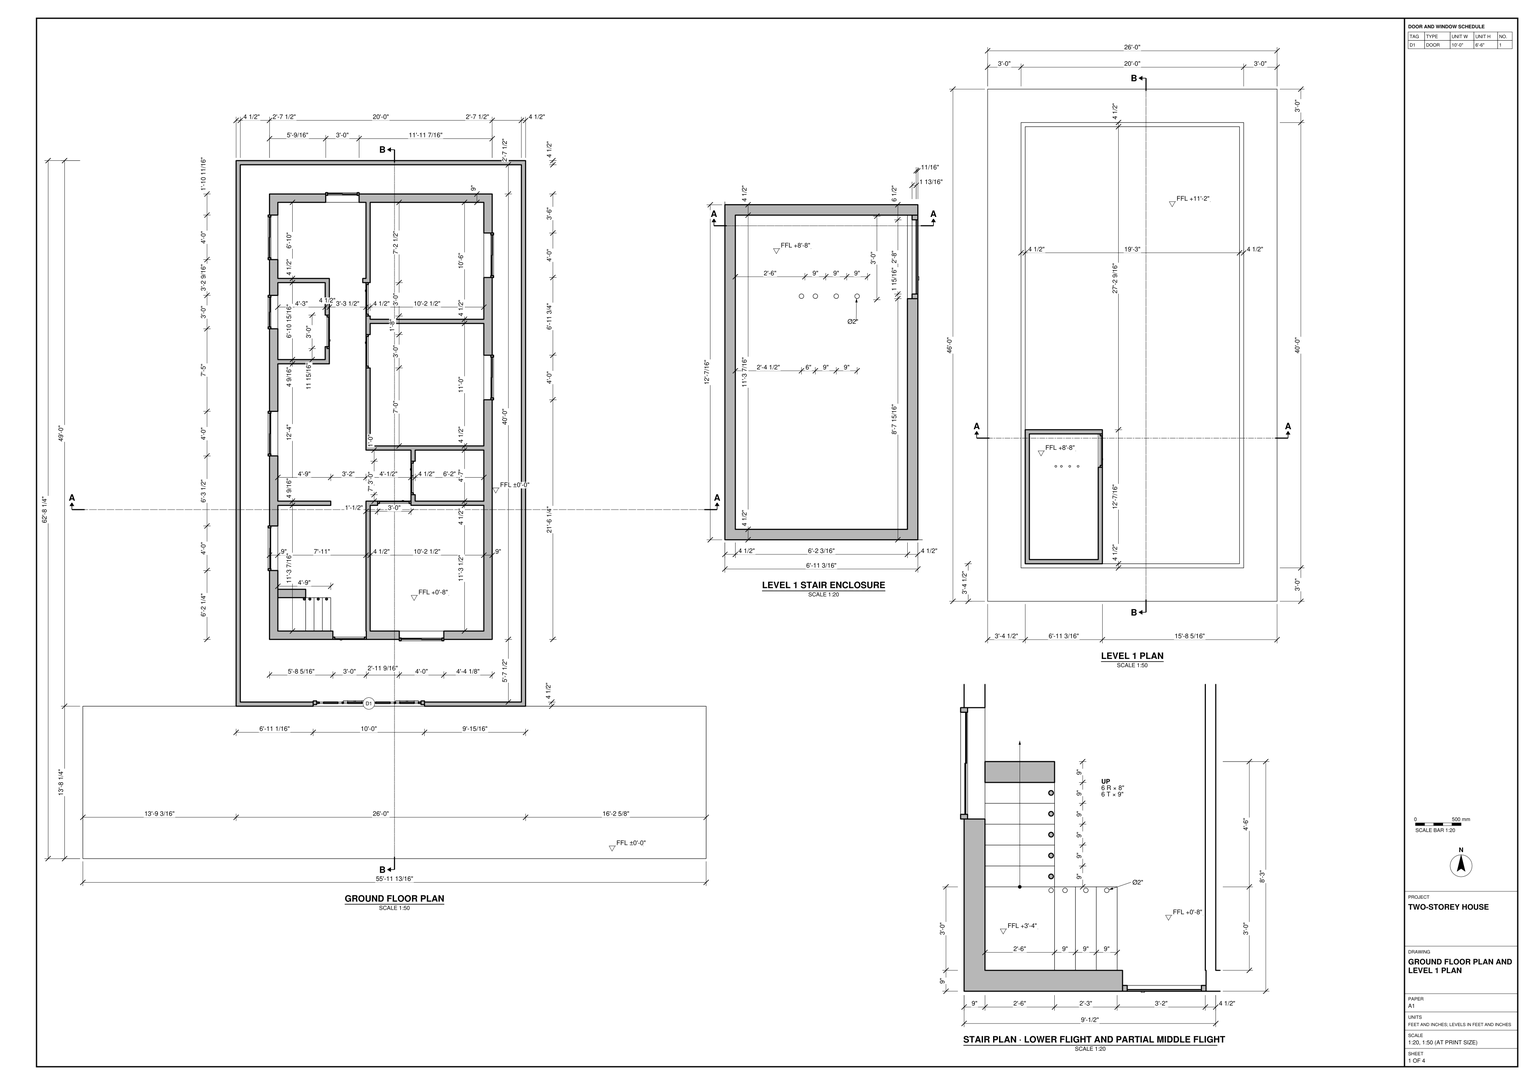
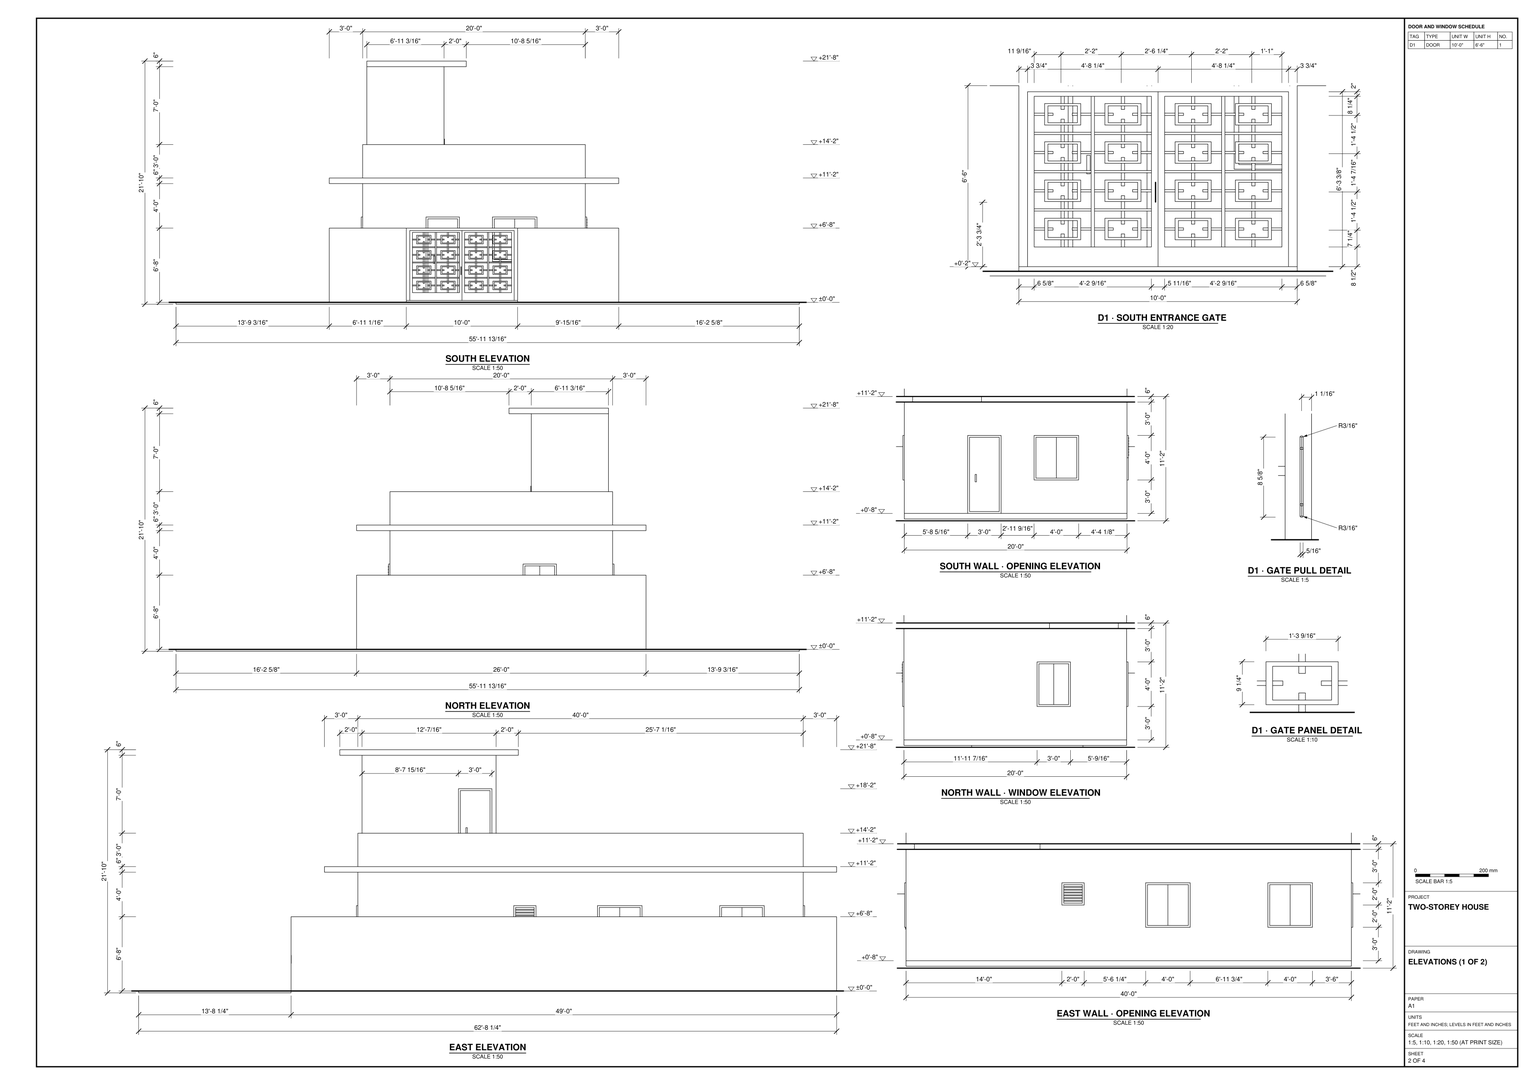
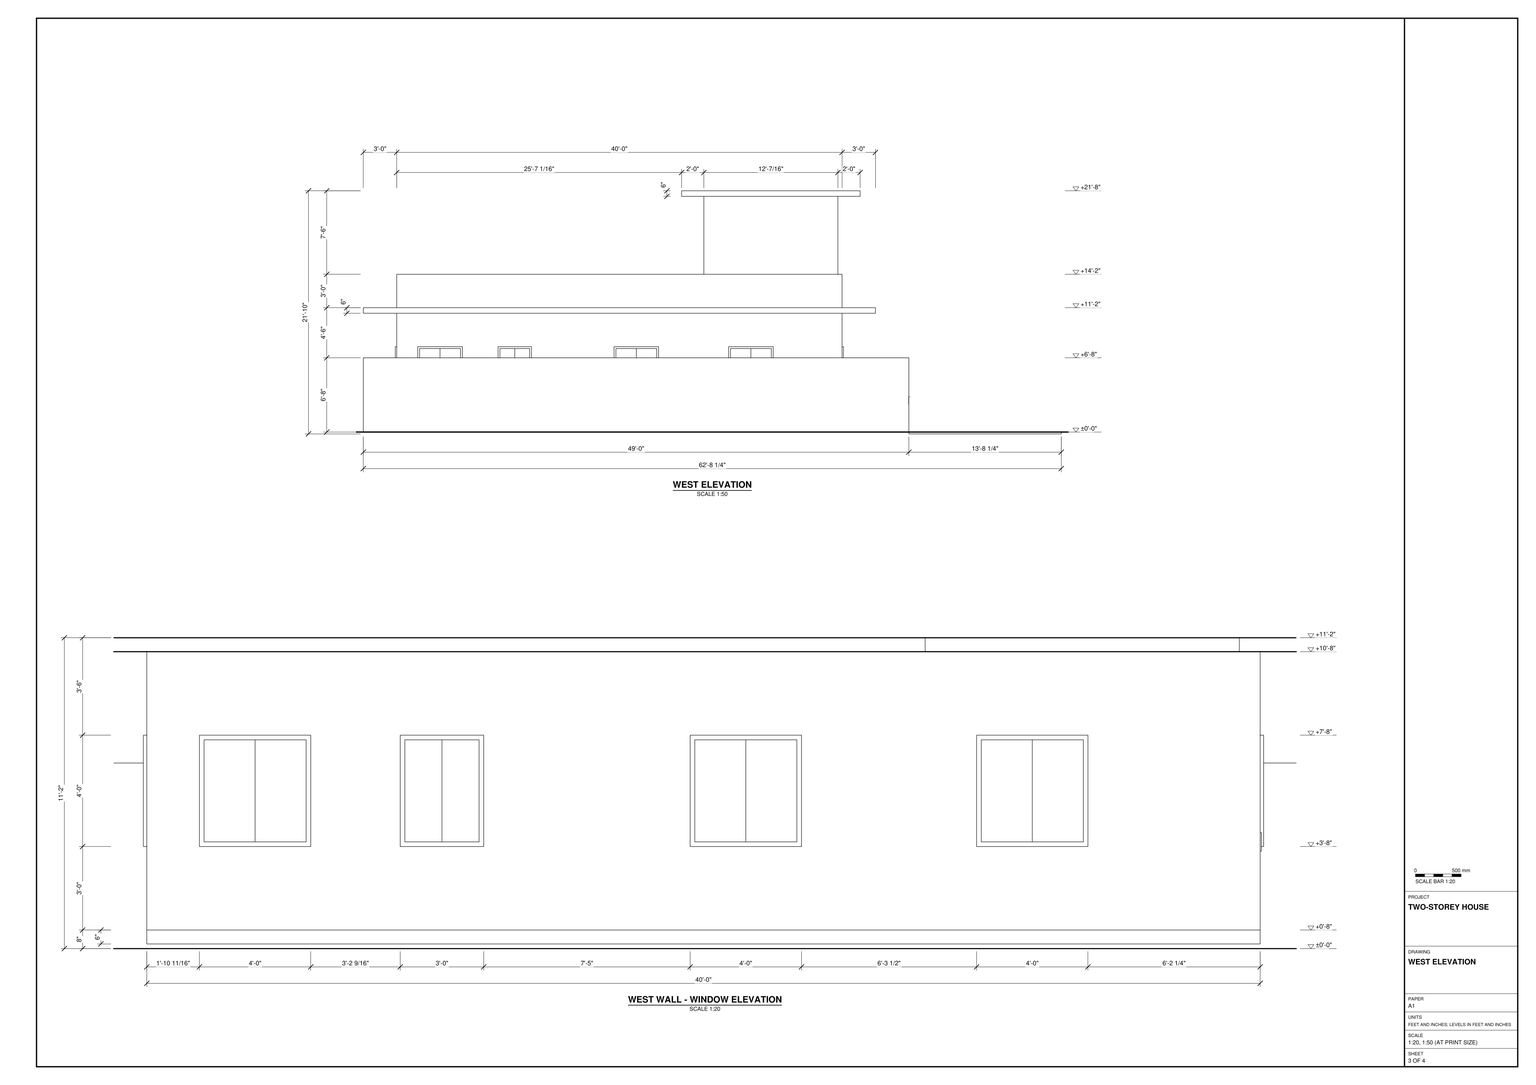
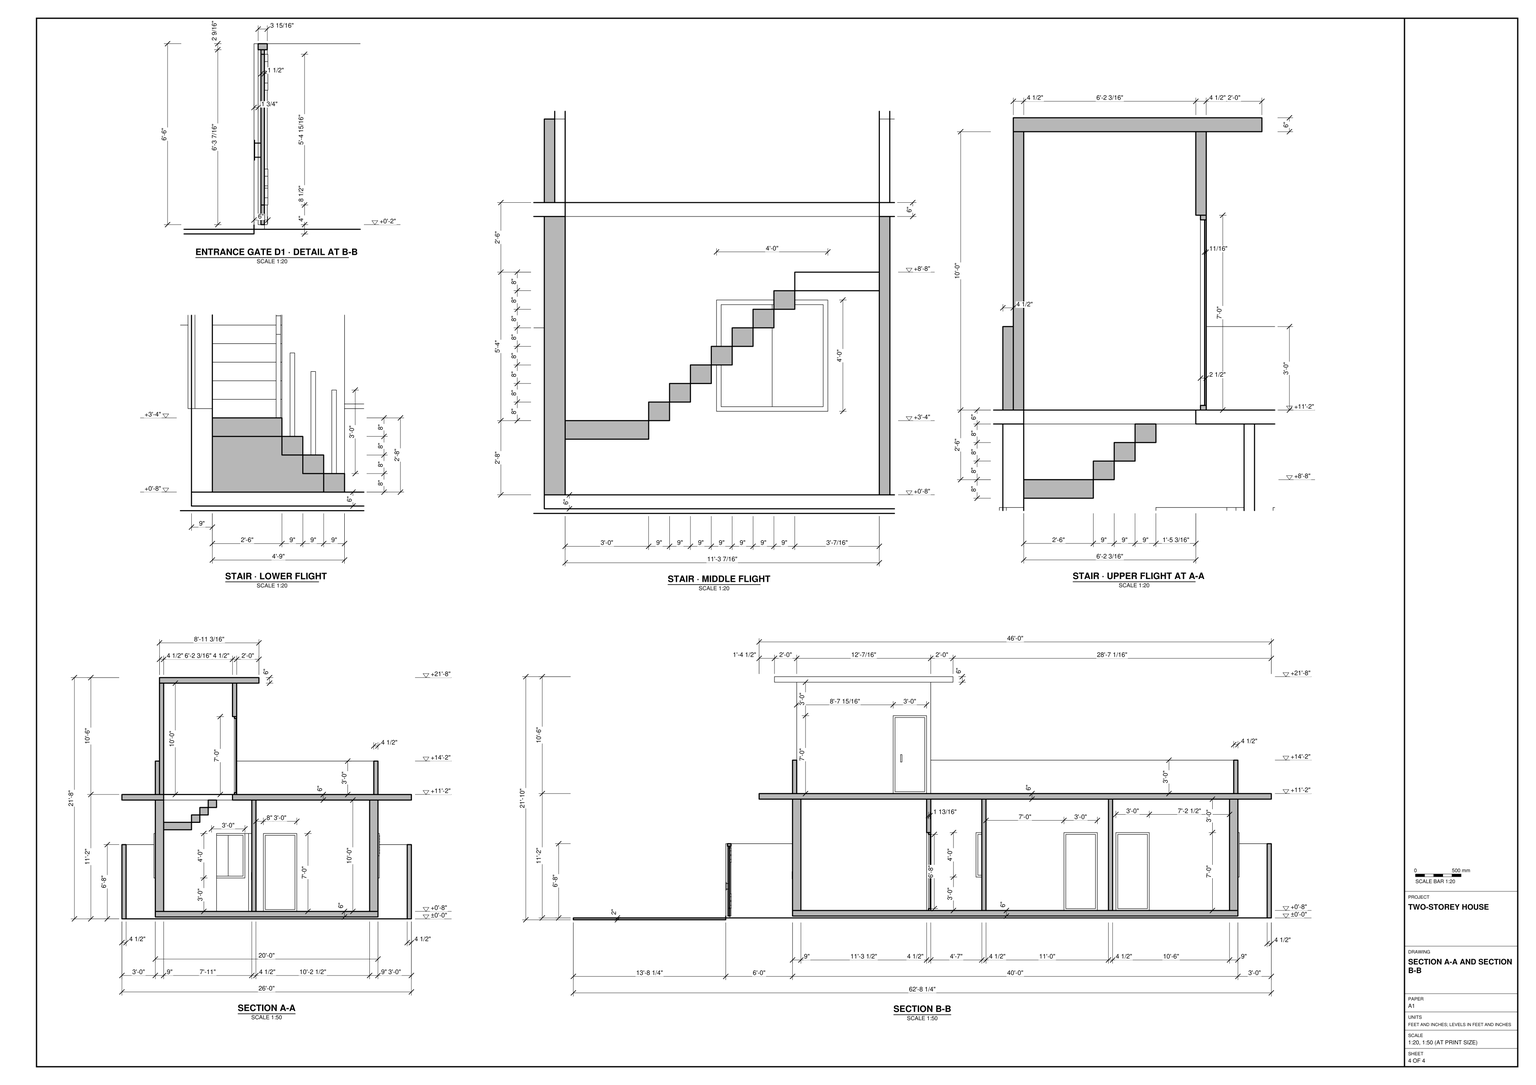
Build the house and its walled site in SketchUp from task_files/diagram_01.pdf. Work in feet and inches. Including the site base, the model measures 55'-11 13/16" east to west, 62'-8 1/4" north to south and 21'-10" high. Use ±0'-0" as the ground datum and +11'-2" as the upper terrace level. Set the interior ground floor above the entrance apron as shown in the elevations.

Lay out the wide apron on the south side, the perimeter wall with its two-leaf entrance gate, and the narrower rectangular house behind it. Follow the ground-floor plan for the exterior wall and partition thicknesses, room layout and circulation. Use the individual wall elevations to place the entrance door, framed windows and vent. Build the turning stair at the southwest corner with its flights and landings. Carry it up through the projecting terrace slab into the roof access enclosure. Include the terrace parapet, the enclosure door and the separate flat roof over the enclosure. Use the enlarged gate detail for the frames, pulls and repeating rectangular panels.

Keep walls, slabs and roofs in separate groups or components, do the same for each furniture or joinery piece shown, and use components for repeated parts. Any decor or loose items shown may be suitable library components. Save one SketchUp model as output_files/two_storey_house_with_a_gated_entrance_and_roof_terrace.skp.

# SketchUp Ruby script. Lengths in inches.
U = 1.inch
M = Sketchup.active_model
def pt(a) = Geom::Point3d.new(a.map { |v| v * U })
def face(e, loops, mat)
  f = e.add_face(loops[0].map { |a| pt(a) })
  loops[1..].each { |l| e.add_face(l.map { |a| pt(a) }).erase! }
  f.material = f.back_material = mat if mat
  f
end
# faces: each face lists its corners as indices into pts; further lists are holes
def faces(e, pts, list, mat = nil) = list.each { |f| face(e, (f[0].is_a?(Array) ? f : [f]).map { |l| l.map { |i| pts[i] } }, mat) }
# xy, xz, yz: faces in a plane at the given z, y or x. An outline is a flat list of corners, or four numbers for a rectangle; further outlines are holes
def ring(l) = l.size == 4 ? [[l[0], l[1]], [l[2], l[1]], [l[2], l[3]], [l[0], l[3]]] : l.each_slice(2).to_a
def flat(e, list, mat, &to3) = list.each { |f| face(e, (f[0].is_a?(Array) ? f : [f]).map { |l| ring(l).map { |u, v| to3.(u, v) } }, mat) }
def xy(e, z, list, mat = nil) = flat(e, list, mat) { |x, y| [x, y, z] }
def xz(e, y, list, mat = nil) = flat(e, list, mat) { |x, z| [x, y, z] }
def yz(e, x, list, mat = nil) = flat(e, list, mat) { |y, z| [x, y, z] }
def lines(e, pts, list) = list.each { |a, b| e.add_line(pt(pts[a]), pt(pts[b])) }
# prism: a flat outline (further loops are holes) pulled along v
def prism(e, loops, v, mat = nil)
  f = face(e, loops, mat); d = Geom::Vector3d.new(v.map { |x| x * U })
  f.pushpull(f.normal.samedirection?(d) ? d.length : -d.length)
end
def box(e, o, s, mat = nil) = prism(e, [[o, [o[0] + s[0], o[1], o[2]], [o[0] + s[0], o[1] + s[1], o[2]], [o[0], o[1] + s[1], o[2]]]], [0, 0, s[2]], mat)
def at(x, y, z, deg = 0) = Geom::Transformation.translation(pt([x, y, z])) * Geom::Transformation.rotation(ORIGIN, Z_AXIS, deg.degrees)
def axes(o, x, y, z) = Geom::Transformation.new([*x, 0, *y, 0, *z, 0, *pt(o).to_a, 1])
def part(name) = M.definitions.add(name)
# library, detail: a bought-in or finely detailed component or shape, given as its bounding box
def library(name, o, s) = part(name).tap { |d| box(d.entities, o, s) }
def detail(e, o, s) = box(e.add_group.entities, o, s)
def put(e, d, t, mat = nil) = e.add_instance(d, t).tap { |i| i.material = mat if mat }
def group(e, t, mat = nil) = e.add_group.tap { |g| g.transformation = t; g.material = mat if mat }.entities
root = M.entities
M.materials.add("Concrete Floor Semigloss 300cm").color = [133, 133, 131]
M.materials.add("Flooring Chevron Light 750cm").color = [151, 128, 98]
M.materials.add("Glass Smoked Distorted 001").color = [38, 38, 38]
M.materials["Glass Smoked Distorted 001"].alpha = 0.1
M.materials.add("Marble Black 100cm").color = [32, 32, 32]
M.materials.add("Marble Emperador Dark 150cm").color = [81, 67, 62]
M.materials.add("Metal Patina 002 180cm").color = [117, 110, 95]
M.materials.add("Tiles K03 100cm").color = [162, 157, 148]
M.materials.add("Wall Paint Bumpy 01 Blue 100cm").color = [86, 103, 109]
M.materials.add("Wall Paint Fine Grain 01 Yellow 100cm").color = [207, 190, 139]
c1 = library("gate 160k",[0,0,0],[125.98,5.98,118.11])
c2 = part("Group\#3")
box(c2.entities,[0,0,0],[22,0.31,44])
c3 = part("Group\#7")
box(c3.entities,[-0.31,0,0],[0.31,22,44])
c4 = part("Group\#9")
box(c4.entities,[-0.31,0,0],[0.31,22,44])
c5 = part("Group\#11")
box(c5.entities,[0,-0.31,0],[16,0.31,44])
c6 = part("Group\#13")
box(c6.entities,[0,0,0],[0.31,22,44])
c7 = part("Group\#15")
box(c7.entities,[0,0,0],[0.3125,16,44])
c8 = part("Group\#17")
box(c8.entities,[0,0,0],[0.31,22,44])
c9 = part("Group\#19")
box(c9.entities,[0,0,0],[0.31,22,44])
c10 = part("Group\#5")
box(c10.entities,[0,0,0],[0.31,20,2])
c11 = library("Group\#45",[0,0,0],[83.6875,144.4375,120])
c12 = library("Group\#39",[0,0,0],[9,36,44])
c13 = library("Group\#42",[0,0,0],[9,36,44])
c14 = library("Group\#52",[-2.5,0,0],[11.5,36,52])
c15 = library("Group\#41",[0,0,0],[30,9,44])
c16 = library("Group\#57",[0,0,0],[30,9,44])
c17 = library("Group\#59",[0,0,0],[30,9,44])
c18 = library("Group\#61",[0,0,0],[30,9,44])
c19 = library("Group\#63",[0,0,0],[30,9,44])
c20 = library("Group\#65",[0,0,0],[30,9,44])
c21 = library("Group\#67",[0,0,0],[30,9,44])
c22 = library("Group\#40",[0,0,0],[30,36.43,44])
c23 = library("Group\#54",[0,0,0],[9,36,44])
c24 = library("Group\#71",[0,0,0],[9,36,44])
c25 = library("Group\#73",[0,0,0],[9,36,44])
put(root,c1,axes([248.25,164.25,-6],[0.9525,0,0],[0,1,0],[0,0,0.6604]))
g1 = group(root,at(201.1875,236.25,0))
xy(g1,0,[[0,0,0,480,240,480,240,0,104.3125,0,104.3125,9,104,9,104,149,116.5,149,116.5,144.5,108.5,144.5,108.5,9,231,9,231,144.5,152.5,144.5,152.5,156,157,156,157,149,231,149,231,204,157,204,157,192,152.5,192,152.5,204,104,204,104,292.5,108.5,292.5,108.5,208.5,231,208.5,231,340.5,108.5,340.5,108.5,328.5,104,328.5,104,348.5,108.5,348.5,108.5,345,231,345,231,471,108.5,471,108.5,384.5,100.5,384.5,100.5,389,104,389,104,471,9,471,9,389,64.5,389,64.5,349.5,60,349.5,60,384.5,9,384.5,9,301.5625,60,301.5625,60,315.5,64.5,315.5,64.5,297,9,297,9,149,66,149,66,144.4375,9,144.4375,9,9,68.3125,9,68.3125,0]])
xy(g1,36,[[139.875,0,187.875,9],[0,74.25,9,122.25],[0,197.75,9,245.75],[231,258.25,240,306.25],[0,334.75,9,370.75],
  [231,390,240,438],[0,409.3125,9,457.3125],[60.5625,471,96.5625,480]])
xy(g1,60,[[231,168,240,192]])
xy(g1,84,[[68.3125,0,104.3125,9],[139.875,0,187.875,9],[0,74.25,9,122.25],[66,144.4375,104,149],[116.5,144.5,152.5,149],
  [152.5,156,157,192],[231,168,240,192],[0,197.75,9,245.75],[231,258.25,240,306.25],[104,292.5,108.5,328.5],
  [60,315.5,64.5,349.5],[0,334.75,9,370.75],[104,348.5,108.5,384.5],[64.5,384.5,100.5,389],[231,390,240,438],
  [0,409.3125,9,457.3125],[60.5625,471,96.5625,480]])
xy(g1,120,[[[0,0,240,480],[9,149,9,297,64.5,297,64.5,384.5,104,384.5,104,204,152.5,204,152.5,149],[108.5,9,231,144.5],[108.5,208.5,231,340.5],[108.5,345,231,471],[9,9,104,144.4375],[9,389,104,471],[9,301.5625,60,384.5],[157,149,231,204]]])
xz(g1,0,[[[0,0,68.3125,0,68.3125,84,104.3125,84,104.3125,0,240,0,240,120,0,120],[139.875,36,187.875,84]]],"Wall Paint Bumpy 01 Blue 100cm")
xz(g1,9,[[9,0,9,120,104,120,104,84,68.3125,84,68.3125,0],[104,0,104.3125,84]])
xz(g1,9,[[[108.5,0,231,120],[139.875,36,187.875,84]]],"Wall Paint Bumpy 01 Blue 100cm")
xz(g1,74.25,[[0,36,9,84]])
xz(g1,122.25,[[0,36,9,84]])
xz(g1,144.4375,[[9,0,66,0,66,84,104,84,104,120,9,120]],"Wall Paint Bumpy 01 Blue 100cm")
xz(g1,144.5,[[108.5,0,116.5,0,116.5,84,152.5,84,152.5,0,231,0,231,120,108.5,120]],"Wall Paint Bumpy 01 Blue 100cm")
xz(g1,149,[[9,0,9,120,152.5,120,152.5,84,116.5,84,116.5,0,104,0,104,84,66,84,66,0],[157,0,231,120]],"Wall Paint Bumpy 01 Blue 100cm")
xz(g1,156,[[152.5,0,157,84]])
xz(g1,168,[[231,60,240,84]])
xz(g1,192,[[152.5,0,157,84],[231,60,240,84]])
xz(g1,197.75,[[0,36,9,84]])
xz(g1,204,[[104,0,152.5,120],[157,0,231,120]],"Wall Paint Bumpy 01 Blue 100cm")
xz(g1,208.5,[[108.5,0,231,120]],"Wall Paint Bumpy 01 Blue 100cm")
xz(g1,245.75,[[0,36,9,84]])
xz(g1,258.25,[[231,36,240,84]])
xz(g1,292.5,[[104,0,108.5,84]])
xz(g1,297,[[9,0,64.5,120]],"Wall Paint Bumpy 01 Blue 100cm")
xz(g1,301.5625,[[9,0,60,120]],"Wall Paint Bumpy 01 Blue 100cm")
xz(g1,306.25,[[231,36,240,84]])
xz(g1,315.5,[[60,0,64.5,84]],"Wall Paint Bumpy 01 Blue 100cm")
xz(g1,328.5,[[104,0,108.5,84]])
xz(g1,334.75,[[0,36,9,84]])
xz(g1,340.5,[[108.5,0,231,120]],"Wall Paint Bumpy 01 Blue 100cm")
xz(g1,345,[[108.5,0,231,120]],"Wall Paint Bumpy 01 Blue 100cm")
xz(g1,348.5,[[104,0,108.5,84]])
xz(g1,349.5,[[60,0,64.5,84]])
xz(g1,370.75,[[0,36,9,84]])
xz(g1,384.5,[[9,0,60,120],[100.5,0,108.5,0,108.5,84,104,84,104,120,64.5,120,64.5,84,100.5,84]],"Wall Paint Bumpy 01 Blue 100cm")
xz(g1,389,[[9,0,9,120,104,120,104,0,100.5,0,100.5,84,64.5,84,64.5,0]],"Wall Paint Bumpy 01 Blue 100cm")
xz(g1,390,[[231,36,240,84]])
xz(g1,409.3125,[[0,36,9,84]])
xz(g1,438,[[231,36,240,84]])
xz(g1,457.3125,[[0,36,9,84]])
xz(g1,471,[[[9,0,104,120],[60.5625,36,96.5625,84]],[108.5,0,231,120]],"Wall Paint Bumpy 01 Blue 100cm")
xz(g1,480,[[[0,0,240,120],[60.5625,36,96.5625,84]]],"Wall Paint Bumpy 01 Blue 100cm")
yz(g1,0,[[[0,0,480,120],[197.75,36,245.75,84],[409.3125,36,457.3125,84],[74.25,36,122.25,84],[334.75,36,370.75,84]]],"Wall Paint Bumpy 01 Blue 100cm")
yz(g1,9,[[[9,0,144.4375,120],[74.25,36,122.25,84]],[[149,0,297,120],[197.75,36,245.75,84]],[[301.5625,0,384.5,120],[334.75,36,370.75,84]],[[389,0,471,120],[409.3125,36,457.3125,84]]],"Wall Paint Bumpy 01 Blue 100cm")
yz(g1,60,[[301.5625,0,301.5625,120,384.5,120,384.5,0,349.5,0,349.5,84,315.5,84,315.5,0]],"Wall Paint Bumpy 01 Blue 100cm")
yz(g1,60.5625,[[471,36,480,84]])
yz(g1,64.5,[[297,0,315.5,0,315.5,84,349.5,84,349.5,0,389,0,389,84,384.5,84,384.5,120,297,120]],"Wall Paint Bumpy 01 Blue 100cm")
yz(g1,66,[[144.4375,0,149,84]])
yz(g1,68.3125,[[0,0,9,84]])
yz(g1,96.5625,[[471,36,480,84]])
yz(g1,100.5,[[384.5,0,389,84]])
yz(g1,104,[[9,0,9,120,144.4375,120,144.4375,84,149,84,149,0],[204,0,204,120,384.5,120,384.5,84,348.5,84,348.5,0,328.5,0,328.5,84,292.5,84,292.5,0],[389,0,471,120]],"Wall Paint Bumpy 01 Blue 100cm")
yz(g1,104.3125,[[0,0,9,84]])
yz(g1,108.5,[[9,0,144.5,120],[208.5,0,292.5,0,292.5,84,328.5,84,328.5,0,340.5,0,340.5,120,208.5,120],[345,0,348.5,0,348.5,84,384.5,84,384.5,0,471,0,471,120,345,120]],"Wall Paint Bumpy 01 Blue 100cm")
yz(g1,116.5,[[144.5,0,149,84]])
yz(g1,139.875,[[0,36,9,84]])
yz(g1,152.5,[[144.5,0,144.5,84,149,84,149,120,204,120,204,0,192,0,192,84,156,84,156,0]],"Wall Paint Bumpy 01 Blue 100cm")
yz(g1,157,[[149,0,156,0,156,84,192,84,192,0,204,0,204,120,149,120]],"Wall Paint Bumpy 01 Blue 100cm")
yz(g1,187.875,[[0,36,9,84]])
yz(g1,231,[[9,0,144.5,120],[[149,0,204,120],[168,60,192,84]],[[208.5,0,340.5,120],[258.25,36,306.25,84]],[[345,0,471,120],[390,36,438,84]]],"Wall Paint Bumpy 01 Blue 100cm")
yz(g1,240,[[[0,0,480,120],[258.25,36,306.25,84],[390,36,438,84],[168,60,192,84]]],"Wall Paint Bumpy 01 Blue 100cm")
g2 = group(g1,at(139.875,0,36))
prism(g2,[[[0,-1.5,0],[48,-1.5,0],[48,-1.5,48],[0,-1.5,48]],[[46,-1.5,46],[46,-1.5,2],[2,-1.5,2],[2,-1.5,46]]],[0,3,0],"Metal Patina 002 180cm")
put(g2,c2,at(2,0.25,2),"Glass Smoked Distorted 001")
put(g2,c2,at(24,-0.06,2),"Glass Smoked Distorted 001")
g3 = group(g1,at(240,258.25,36))
prism(g3,[[[1.5,0,0],[1.5,48,0],[1.5,48,48],[1.5,0,48]],[[1.5,2,2],[1.5,2,46],[1.5,46,46],[1.5,46,2]]],[-3,0,0])
put(g3,c3,at(-0.3125,2,2))
put(g3,c3,at(0,24,2))
g4 = group(g1,at(240,390,36))
prism(g4,[[[1.5,48,0],[1.5,48,48],[1.5,0,48],[1.5,0,0]],[[1.5,46,2],[1.5,2,2],[1.5,2,46],[1.5,46,46]]],[-3,0,0])
put(g4,c4,at(-0.1875,2,2))
put(g4,c4,at(0.13,24,2))
g5 = group(g1,at(60.5625,480,36))
prism(g5,[[[36,1.5,0],[0,1.5,0],[0,1.5,48],[36,1.5,48]],[[34,1.5,2],[34,1.5,46],[2,1.5,46],[2,1.5,2]]],[0,-3,0],"Metal Patina 002 180cm")
put(g5,c5,at(18,0,2),"Glass Smoked Distorted 001")
put(g5,c5,at(2,0.31,2),"Glass Smoked Distorted 001")
g6 = group(g1,at(0,409.3125,36))
prism(g6,[[[-1.5,0,0],[-1.5,0,48],[-1.5,48,48],[-1.5,48,0]],[[-1.5,46,46],[-1.5,2,46],[-1.5,2,2],[-1.5,46,2]]],[3,0,0],"Metal Patina 002 180cm")
put(g6,c6,at(0.0625,24,2),"Glass Smoked Distorted 001")
put(g6,c6,at(-0.25,2,2),"Glass Smoked Distorted 001")
g7 = group(g1,at(0,334.75,36))
prism(g7,[[[-1.5,0,0],[-1.5,0,48],[-1.5,36,48],[-1.5,36,0]],[[-1.5,2,46],[-1.5,2,2],[-1.5,34,2],[-1.5,34,46]]],[3,0,0],"Metal Patina 002 180cm")
put(g7,c7,at(0.25,18,2),"Glass Smoked Distorted 001")
put(g7,c7,at(-0.0625,2,2),"Glass Smoked Distorted 001")
g8 = group(g1,at(0,197.75,36))
prism(g8,[[[-1.5,48,0],[-1.5,0,0],[-1.5,0,48],[-1.5,48,48]],[[-1.5,46,2],[-1.5,46,46],[-1.5,2,46],[-1.5,2,2]]],[3,0,0],"Metal Patina 002 180cm")
put(g8,c8,at(0.4375,24,2),"Glass Smoked Distorted 001")
put(g8,c8,at(0.12,2,2),"Glass Smoked Distorted 001")
g9 = group(g1,at(0,74.25,36))
prism(g9,[[[-1.5,48,0],[-1.5,0,0],[-1.5,0,48],[-1.5,48,48]],[[-1.5,2,2],[-1.5,46,2],[-1.5,46,46],[-1.5,2,46]]],[3,0,0],"Metal Patina 002 180cm")
put(g9,c9,at(0.6875,24,2),"Glass Smoked Distorted 001")
put(g9,c9,at(0.37,2,2),"Glass Smoked Distorted 001")
g10 = group(g1,at(68.3125,0,0))
prism(g10,[[[36,0,0],[36,0,84],[0,0,84],[0,0,0]],[[2,0,82],[34,0,82],[34,0,2],[2,0,2]]],[0,2.5,0],"Metal Patina 002 180cm")
g11 = group(g10,at(2,0,2))
box(g11,[0,0,0],[32,0.71,80],"Flooring Chevron Light 750cm")
g12 = group(g11,at(6,0,32),"Metal Patina 002 180cm")
xy(g12,0,[[0,-0.5,1.5,0]])
xy(g12,8,[[0,-0.5,1.5,0]])
xz(g12,-0.5,[[0,0,1.5,8]],"Metal Patina 002 180cm")
xz(g12,0,[[0,0,1.5,8]],"Metal Patina 002 180cm")
yz(g12,0,[[-0.5,0,0,8]])
yz(g12,1.5,[[-0.5,0,0,8]])
g13 = group(g1,at(64.5,313.5,0))
prism(g13,[[[0,36,0],[0,36,84],[0,0,84],[0,0,0]],[[0,34,82],[0,34,2],[0,2,2],[0,2,82]]],[-2.5,0,0],"Metal Patina 002 180cm")
g14 = group(g13,at(0,2,2))
box(g14,[-0.71,0,0],[0.71,32,80],"Flooring Chevron Light 750cm")
g15 = group(g14,at(0,6,32),"Metal Patina 002 180cm")
box(g15,[0,0,0],[0.5,1.5,8])
g16 = group(g1,at(104,348.5,0))
prism(g16,[[[0,0,0],[0,0,84],[0,36,84],[0,36,0]],[[0,2,82],[0,2,2],[0,34,2],[0,34,82]]],[2.5,0,0],"Metal Patina 002 180cm")
g17 = group(g16,at(0,2,2))
box(g17,[0,0,0],[0.71,32,80],"Flooring Chevron Light 750cm")
g18 = group(g17,at(0,26,32),"Metal Patina 002 180cm")
box(g18,[-0.5,-1.5,0],[0.5,1.5,8])
g19 = group(g1,at(104,292.5,0))
prism(g19,[[[0,0,0],[0,0,84],[0,36,84],[0,36,0]],[[0,34,82],[0,2,82],[0,2,2],[0,34,2]]],[2.5,0,0],"Metal Patina 002 180cm")
g20 = group(g19,at(0,2,2))
box(g20,[0,0,0],[0.71,32,80],"Flooring Chevron Light 750cm")
g21 = group(g20,at(0,26,32),"Metal Patina 002 180cm")
box(g21,[-0.5,-1.5,0],[0.5,1.5,8])
g22 = group(g1,at(152.5,156,0))
prism(g22,[[[0,0,0],[0,0,84],[0,36,84],[0,36,0]],[[0,34,82],[0,2,82],[0,2,2],[0,34,2]]],[2.5,0,0],"Metal Patina 002 180cm")
g23 = group(g22,at(0,2,2))
box(g23,[0,0,0],[0.71,32,80],"Flooring Chevron Light 750cm")
g24 = group(g23,at(0,26,32),"Metal Patina 002 180cm")
box(g24,[-0.5,-1.5,0],[0.5,1.5,8])
g25 = group(g1,at(116.5,149,0))
prism(g25,[[[0,0,0],[0,0,84],[36,0,84],[36,0,0]],[[34,0,2],[34,0,82],[2,0,82],[2,0,2]]],[0,-2.5,0],"Metal Patina 002 180cm")
g26 = group(g25,at(2,0,2))
box(g26,[0,-0.71,0],[32,0.71,80],"Flooring Chevron Light 750cm")
g27 = group(g26,at(26,0,32),"Metal Patina 002 180cm")
box(g27,[-1.5,0,0],[1.5,0.5,8])
g28 = group(g1,at(240,168,60))
prism(g28,[[[1.5,0,0],[1.5,24,0],[1.5,24,24],[1.5,0,24]],[[1.5,22,22],[1.5,22,2],[1.5,2,2],[1.5,2,22]]],[-3,0,0])
put(g28,c10,at(1.5,2,20))
put(g28,c10,at(1.5,2,17))
put(g28,c10,at(1.5,2,14))
put(g28,c10,at(1.5,2,11))
put(g28,c10,at(1.5,2,8))
put(g28,c10,at(1.5,2,5))
put(g28,c10,at(1.5,2,2))
g29 = group(root,at(201.1875,236.25,120))
xy(g29,0,[[[-36,-36,276,516],[9,9,83.1875,144.4375]]],"Marble Black 100cm")
xy(g29,6,[[[-36,-36,276,516],[4.5,4.5,87.6875,148.9375]]],"Marble Black 100cm")
xz(g29,-36,[[-36,0,276,6]],"Marble Black 100cm")
xz(g29,9,[[9,0,83.1875,6]],"Marble Black 100cm")
xz(g29,144.4375,[[9,0,83.1875,6]],"Marble Black 100cm")
xz(g29,516,[[-36,0,276,6]],"Marble Black 100cm")
yz(g29,-36,[[-36,0,516,6]],"Marble Black 100cm")
yz(g29,9,[[9,0,144.4375,6]],"Marble Black 100cm")
yz(g29,83.1875,[[9,0,144.4375,6]],"Marble Black 100cm")
yz(g29,276,[[-36,0,516,6]],"Marble Black 100cm")
g30 = group(g29,at(0,0,6),"Wall Paint Fine Grain 01 Yellow 100cm")
prism(g30,[[[240,0,0],[0,0,0],[0,480,0],[240,480,0]],[[4.5,475.5,0],[4.5,4.5,0],[235.5,4.5,0],[235.5,475.5,0]]],[0,0,36],"Wall Paint Fine Grain 01 Yellow 100cm")
put(g29,c11,at(4.5,4.5,6))
g31 = group(g29,at(4.5,4.5,126),"Wall Paint Fine Grain 01 Yellow 100cm")
box(g31,[0,-24,0],[107.1875,192.4375,6],"Wall Paint Fine Grain 01 Yellow 100cm")
put(root,c12,at(258.1875,245.25,0))
g32 = group(root,at(201.1875,236.25,-6),"Marble Black 100cm")
box(g32,[0,0,0],[240,480,6],"Marble Black 100cm")
put(root,c13,at(249.1875,245.25,8))
put(root,c14,at(240.1875,245.25,16))
g33 = group(root,at(231.1875,245.25,24))
box(g33,[-21,0,0],[30,36,8],"Marble Emperador Dark 150cm")
put(root,c15,at(210.1875,281.25,32))
put(root,c16,at(210.1875,290.25,40))
put(root,c17,at(210.1875,299.25,48))
put(root,c18,at(210.1875,308.25,56))
put(root,c19,at(210.1875,317.25,64))
put(root,c20,at(210.1875,326.25,72))
put(root,c21,at(210.1875,335.25,80))
put(root,c22,at(210.1875,344.25,88))
put(root,c23,at(240.1875,344.25,96))
put(root,c24,at(249.1875,344.25,104))
put(root,c25,at(258.1875,344.25,112))
g34 = group(root,at(165.1875,164.25,-6))
g35 = group(g34,at(0,0,0))
xy(g35,-2,[[83.0625,0,203.0625,0,203.0625,4.5,307.5,4.5,307.5,583.5,4.5,583.5,4.5,4.5,83.0625,4.5]],"Tiles K03 100cm")
xy(g35,-2,[[0,0,83.0625,0,83.0625,4.5,4.5,4.5,4.5,583.5,307.5,583.5,307.5,4.5,203.0625,4.5,203.0625,0,312,0,312,588,0,588]],"Wall Paint Fine Grain 01 Yellow 100cm")
xy(g35,78,[[0,0,83.0625,0,83.0625,4.5,4.5,4.5,4.5,583.5,307.5,583.5,307.5,4.5,203.0625,4.5,203.0625,0,312,0,312,588,0,588]],"Wall Paint Fine Grain 01 Yellow 100cm")
xz(g35,0,[[0,-2,83.0625,78],[83.0625,-2,203.0625,0],[203.0625,-2,312,78]],"Wall Paint Fine Grain 01 Yellow 100cm")
xz(g35,4.5,[[4.5,-2,83.0625,78],[203.0625,-2,307.5,78]],"Wall Paint Fine Grain 01 Yellow 100cm")
xz(g35,583.5,[[4.5,-2,307.5,78]],"Wall Paint Fine Grain 01 Yellow 100cm")
xz(g35,588,[[0,-2,312,78]],"Wall Paint Fine Grain 01 Yellow 100cm")
yz(g35,0,[[0,-2,588,78]],"Wall Paint Fine Grain 01 Yellow 100cm")
yz(g35,4.5,[[4.5,-2,583.5,78]],"Wall Paint Fine Grain 01 Yellow 100cm")
yz(g35,83.0625,[[0,-2,4.5,78]],"Wall Paint Fine Grain 01 Yellow 100cm")
yz(g35,203.0625,[[0,-2,4.5,78]],"Wall Paint Fine Grain 01 Yellow 100cm")
yz(g35,307.5,[[4.5,-2,583.5,78]],"Wall Paint Fine Grain 01 Yellow 100cm")
yz(g35,312,[[0,-2,588,78]],"Wall Paint Fine Grain 01 Yellow 100cm")
g36 = group(root,at(165.1875,99.625,-8))
box(g36,[-165.1875,-99.625,-2],[671.8125,164.25,2],"Concrete Floor Semigloss 300cm")
